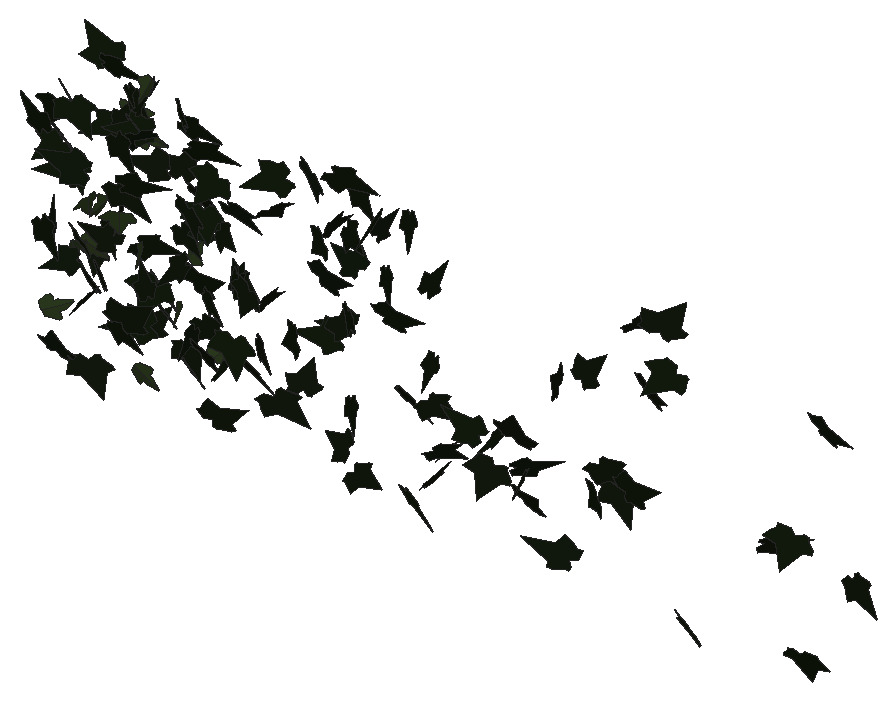
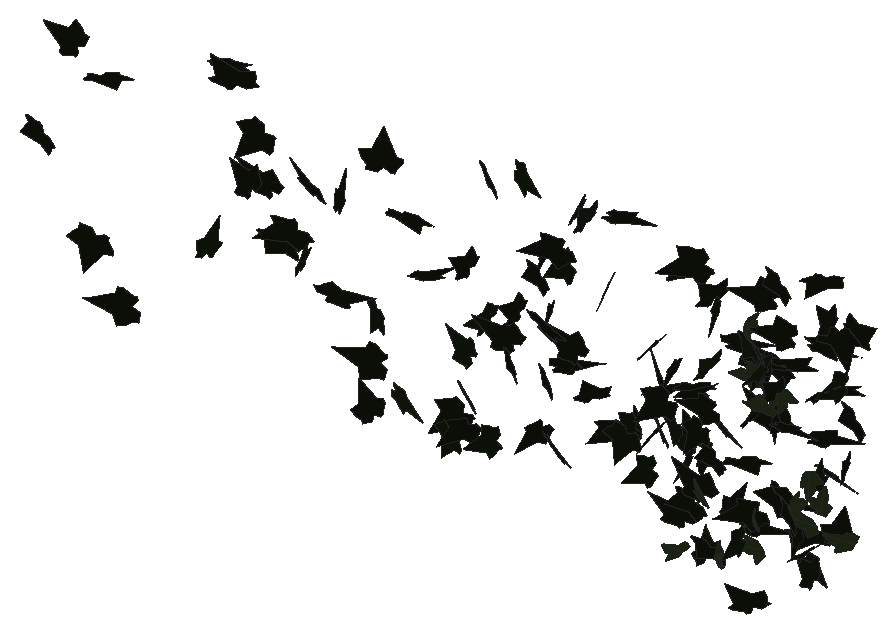
# SketchUp Ruby script. Lengths in inches.
U = 1.inch
M = Sketchup.active_model
def pt(a) = Geom::Point3d.new(a.map { |v| v * U })
def face(e, loops, mat)
  f = e.add_face(loops[0].map { |a| pt(a) })
  loops[1..].each { |l| e.add_face(l.map { |a| pt(a) }).erase! }
  f.material = f.back_material = mat if mat
  f
end
# faces: each face lists its corners as indices into pts; further lists are holes
def faces(e, pts, list, mat = nil) = list.each { |f| face(e, (f[0].is_a?(Array) ? f : [f]).map { |l| l.map { |i| pts[i] } }, mat) }
# xy, xz, yz: faces in a plane at the given z, y or x. An outline is a flat list of corners, or four numbers for a rectangle; further outlines are holes
def ring(l) = l.size == 4 ? [[l[0], l[1]], [l[2], l[1]], [l[2], l[3]], [l[0], l[3]]] : l.each_slice(2).to_a
def flat(e, list, mat, &to3) = list.each { |f| face(e, (f[0].is_a?(Array) ? f : [f]).map { |l| ring(l).map { |u, v| to3.(u, v) } }, mat) }
def xy(e, z, list, mat = nil) = flat(e, list, mat) { |x, y| [x, y, z] }
def xz(e, y, list, mat = nil) = flat(e, list, mat) { |x, z| [x, y, z] }
def yz(e, x, list, mat = nil) = flat(e, list, mat) { |y, z| [x, y, z] }
def lines(e, pts, list) = list.each { |a, b| e.add_line(pt(pts[a]), pt(pts[b])) }
# prism: a flat outline (further loops are holes) pulled along v
def prism(e, loops, v, mat = nil)
  f = face(e, loops, mat); d = Geom::Vector3d.new(v.map { |x| x * U })
  f.pushpull(f.normal.samedirection?(d) ? d.length : -d.length)
end
def box(e, o, s, mat = nil) = prism(e, [[o, [o[0] + s[0], o[1], o[2]], [o[0] + s[0], o[1] + s[1], o[2]], [o[0], o[1] + s[1], o[2]]]], [0, 0, s[2]], mat)
def at(x, y, z, deg = 0) = Geom::Transformation.translation(pt([x, y, z])) * Geom::Transformation.rotation(ORIGIN, Z_AXIS, deg.degrees)
def axes(o, x, y, z) = Geom::Transformation.new([*x, 0, *y, 0, *z, 0, *pt(o).to_a, 1])
def part(name) = M.definitions.add(name)
# library, detail: a bought-in or finely detailed component or shape, given as its bounding box
def library(name, o, s) = part(name).tap { |d| box(d.entities, o, s) }
def detail(e, o, s) = box(e.add_group.entities, o, s)
def put(e, d, t, mat = nil) = e.add_instance(d, t).tap { |i| i.material = mat if mat }
def group(e, t, mat = nil) = e.add_group.tap { |g| g.transformation = t; g.material = mat if mat }.entities
root = M.entities
M.materials.add("1026 AP 7946 SUNNY SIDE UP").color = [254, 231, 186]
M.materials.add("efeu1").color = [18, 25, 13]
M.materials.add("efeu2").color = [43, 57, 29]
c1 = part("ivyleaf_9")
p = [[1.54,2.16,1.25],[1.36,2.04,1.19],[-0.21,0.99,0.68],[-0.71,1.11,0.82],[-0.85,0.86,0.67],[-0.8,0.17,0.21],
  [-0.9,-0.01,0.1],[-0.67,-0.16,-0.02],[-0.08,-0.08,-0.05],[-0.03,-0.6,-0.4],[0.65,-0.88,-0.66],[0.83,-0.6,-0.49],
  [1.29,-0.42,-0.43],[1.8125,-0.07,-0.26],[1.21,0.44,0.15]]
faces(c1.entities,p,[[0,1,2,3,4,5,6,7,8,9,10,11,12,13,14]],"efeu1")
c2 = part("ivyleaf_10")
p = [[0,0.5,-0.03],[-0.0625,2.02,-0.43],[-0.19,2.01,-0.46],[-0.54,1.05,-0.29],[-0.52,0.625,-0.18],[-0.83,0.76,-0.28],
  [-1.16,0.64,-0.33],[-1.15,0.33,-0.24],[-0.77,-0.39,0.02],[-0.3,-0.51,0.16],[0.04,-0.48,0.23],[-0.02,2.01,-0.4375],
  [-0.06,2.01,-0.43],[0.04,-0.49,0.23],[0.67,-0.49,0.14],[1.38,0.36,-0.2],[1.375,0.51,-0.24],[0.81,0.65,-0.19],
  [0.62,0.59,-0.15],[0.6,1.09,-0.28],[0.5,1.23,-0.31]]
faces(c2.entities,p,[[0,1,2,3,4,5,6,7,8,9,10],[11,12,0,13,14,15,16,17,18,19,20]],"efeu2")
put(root,c1,axes([156.98,210.53,286.43],[-0.47696,-0.0723,0.34945],[-0.49379,-0.13528,-0.31941],[0.23295,-0.4348,0.03841]),"1026 AP 7946 SUNNY SIDE UP")
put(root,c1,axes([156.96,212.43,290.43],[-0.65372,-0.19497,-0.00524],[-0.03193,0.03396,0.47151],[-0.30497,0.41438,-0.03813]),"1026 AP 7946 SUNNY SIDE UP")
put(root,c1,axes([156.29,211.76,281.18],[0.15068,-0.21401,0.39414],[0.19777,-0.36304,-0.24301],[0.66207,0.15715,-0.01711]),"1026 AP 7946 SUNNY SIDE UP")
put(root,c1,axes([156.55,212.05,282.28],[-0.09183,-0.37678,0.07217],[-0.00305,-0.07274,-0.39311],[0.60323,-0.05773,0.009]),"1026 AP 7946 SUNNY SIDE UP")
put(root,c1,axes([156.81,209.09,284.39],[-0.06746,-0.14859,0.41575],[0.1899,0.38597,0.16155],[-0.65029,0.12813,0.00405]),"1026 AP 7946 SUNNY SIDE UP")
put(root,c1,axes([156.93,209.47,288.05],[-0.43996,-0.22259,0.17657],[-0.16855,-0.14092,-0.36694],[0.40962,-0.29705,0.03866]),"1026 AP 7946 SUNNY SIDE UP")
put(root,c1,axes([156.47,209.7,288.51],[0.53514,-0.28084,0.00143],[-0.02885,-0.0269,-0.45349],[0.44068,0.33928,-0.03142]),"1026 AP 7946 SUNNY SIDE UP")
put(root,c2,axes([156.85,212.1,284.22],[0.05882,-0.06243,0.38985],[0.14433,-0.36808,-0.07399],[0.58612,0.0969,-0.0209]),"1026 AP 7946 SUNNY SIDE UP")
put(root,c1,axes([157.3,212.36,287.67],[-0.55836,-0.03377,0.15532],[-0.22596,-0.06788,-0.36428],[0.09002,-0.37984,0.04898]),"1026 AP 7946 SUNNY SIDE UP")
put(root,c2,axes([157.02,211.03,284.94],[-0.12068,-0.38239,-0.10532],[0.04398,0.09642,-0.40114],[0.61995,-0.08127,0.00796]),"1026 AP 7946 SUNNY SIDE UP")
put(root,c1,axes([157.3,207.87,289.59],[0.10643,-0.08708,0.41704],[-0.33907,0.34336,0.1151],[-0.55673,-0.22576,0.00963]),"1026 AP 7946 SUNNY SIDE UP")
put(root,c1,axes([157.29,208.88,290.14],[0.45969,0.1171,-0.34721],[-0.46,-0.17227,-0.32345],[-0.32291,0.41211,-0.03352]),"1026 AP 7946 SUNNY SIDE UP")
put(root,c2,axes([157.16,210.14,283.16],[-0.15146,-0.31849,-0.23263],[-0.05871,-0.22214,0.34061],[-0.60943,0.10055,0.025]),"1026 AP 7946 SUNNY SIDE UP")
put(root,c1,axes([157.4,210.64,281.125],[-0.2473,0.28417,-0.22099],[0.13859,-0.19795,-0.33537],[-0.54401,-0.17961,0.01502]),"1026 AP 7946 SUNNY SIDE UP")
put(root,c2,axes([156.89,208.78,281.2],[0.21959,0.05592,-0.3699],[0.47428,0.19729,0.15353],[0.31955,-0.33125,0.02632]),"1026 AP 7946 SUNNY SIDE UP")
put(root,c2,axes([156.9,211.125,283],[-0.15781,-0.00986,-0.38759],[0.53061,-0.17465,-0.08905],[-0.26185,-0.34796,0.05313]),"1026 AP 7946 SUNNY SIDE UP")
put(root,c1,axes([157.32,211.83,283.62],[-0.15407,-0.05736,-0.45334],[0.68366,-0.10099,-0.08683],[-0.13713,-0.43904,0.07645]),"1026 AP 7946 SUNNY SIDE UP")
put(root,c1,axes([157.5,209.95,283.87],[0.40486,-0.27997,-0.16395],[0.22451,-0.08114,0.38846],[-0.45252,-0.29074,0.04605]),"1026 AP 7946 SUNNY SIDE UP")
put(root,c1,axes([157.8,210.69,282.3],[0.38912,-0.12408,-0.28524],[-0.42309,0.07341,-0.28193],[0.21828,0.36349,-0.03797]),"1026 AP 7946 SUNNY SIDE UP")
put(root,c1,axes([158.3,210.9,283.57],[-0.24504,0.13816,0.36682],[-0.46789,0.19583,-0.21176],[-0.37467,-0.33491,0.02455]),"1026 AP 7946 SUNNY SIDE UP")
put(root,c1,axes([158.27,208.62,283.81],[-0.58292,0.12185,0.08032],[-0.13464,-0.01432,-0.40003],[-0.18261,-0.37842,0.03855]),"1026 AP 7946 SUNNY SIDE UP")
put(root,c1,axes([157.56,209.14,290.48],[0.1385,-0.2344,0.36129],[0.14402,-0.34048,-0.25916],[0.64924,0.12553,-0.01958]),"1026 AP 7946 SUNNY SIDE UP")
put(root,c1,axes([157.77,209.3,287.59],[0.00105,-0.38969,-0.05874],[0.00218,0.0548,-0.40113],[0.61877,0.00047,0.00151]),"1026 AP 7946 SUNNY SIDE UP")
put(root,c2,axes([157.92,212.68,288.28],[0.61115,0.04956,-0.01353],[0.01222,0.04445,0.40146],[0.07981,-0.38636,0.04213]),"1026 AP 7946 SUNNY SIDE UP")
put(root,c1,axes([157.64,207.5,285.67],[-0.13472,-0.06788,-0.47571],[0.73317,-0.02084,-0.08616],[-0.01308,-0.4688,0.0699]),"1026 AP 7946 SUNNY SIDE UP")
put(root,c1,axes([158.23,211.51,288.37],[-0.15955,-0.07341,0.3889],[0.37642,0.29405,0.12678],[-0.47409,0.25818,-0.03022]),"1026 AP 7946 SUNNY SIDE UP")
put(root,c1,axes([158.22,207.64,280.35],[0.57197,-0.16928,0.12798],[-0.14963,0.09076,0.41178],[-0.29532,-0.37384,0.03925]),"1026 AP 7946 SUNNY SIDE UP")
put(root,c1,axes([157.77,211.34,290.89],[0.43355,-0.07208,0.29989],[0.41706,-0.12708,-0.29157],[0.22137,0.38059,-0.038]),"1026 AP 7946 SUNNY SIDE UP")
put(root,c1,axes([158.36,211.95,289.65],[0.45232,-0.35053,-0.09835],[-0.12695,0.05445,-0.46598],[0.55613,0.29753,-0.02638]),"1026 AP 7946 SUNNY SIDE UP")
put(root,c1,axes([159.29,207.76,288.46],[-0.44169,-0.17637,-0.35042],[-0.48797,-0.14052,0.33927],[-0.35096,0.41735,-0.0307]),"1026 AP 7946 SUNNY SIDE UP")
put(root,c2,axes([158.8125,212,283.01],[0.12533,-0.17766,0.35121],[0.26866,-0.29666,-0.20157],[0.54306,0.18777,0.01866]),"1026 AP 7946 SUNNY SIDE UP")
put(root,c1,axes([158.76,212.26,279.35],[-0.24949,-0.02099,0.41106],[0.61229,0.08869,0.16479],[-0.14167,0.42026,-0.01167]),"1026 AP 7946 SUNNY SIDE UP")
put(root,c1,axes([158.99,211.34,289.44],[-0.09333,0.32331,0.26054],[0.09219,-0.24437,0.33703],[0.63702,0.08273,-0.0106]),"1026 AP 7946 SUNNY SIDE UP")
put(root,c1,axes([158.87,211.97,283.25],[0.09768,0.09358,-0.42869],[0.1525,0.40694,0.11143],[0.65392,-0.10888,0.03805]),"1026 AP 7946 SUNNY SIDE UP")
put(root,c1,axes([159.03,207.58,291.3],[-0.11704,-0.34068,-0.2994],[0.13206,0.27677,-0.35716],[0.68961,-0.11082,0.01758]),"1026 AP 7946 SUNNY SIDE UP")
put(root,c1,axes([159.55,211.47,290.08],[-0.30208,0.18477,-0.35045],[-0.3728,0.24553,0.27592],[0.48302,0.30506,-0.00622]),"1026 AP 7946 SUNNY SIDE UP")
put(root,c1,axes([159.29,210.91,289.05],[0.50554,-0.04998,-0.26158],[-0.37961,0.08667,-0.33236],[0.14533,0.40023,0.04179]),"1026 AP 7946 SUNNY SIDE UP")
put(root,c1,axes([159.87,210.94,288.9],[-0.46343,0.0187,0.29618],[-0.44927,-0.07063,-0.29754],[0.05688,-0.40555,0.06303]),"1026 AP 7946 SUNNY SIDE UP")
put(root,c1,axes([159.47,210.08,286.16],[-0.17716,0.05385,-0.46499],[0.55483,-0.28329,-0.12713],[-0.45134,-0.36938,0.02623]),"1026 AP 7946 SUNNY SIDE UP")
put(root,c1,axes([159.43,212.09,281.89],[0.53175,-0.23609,-0.13661],[-0.20248,0.04399,-0.42301],[0.37337,0.36008,-0.03485]),"1026 AP 7946 SUNNY SIDE UP")
put(root,c1,axes([159.81,210.46,288.9375],[0.20341,0.36905,-0.12404],[-0.04412,-0.11991,-0.40336],[-0.60983,0.13177,-0.01219]),"1026 AP 7946 SUNNY SIDE UP")
put(root,c2,axes([159.68,211.34,290.71],[-0.05764,-0.21073,0.35169],[0.18287,-0.33486,-0.20134],[0.60541,0.08108,0.0943]),"1026 AP 7946 SUNNY SIDE UP")
put(root,c1,axes([159.625,207.84,280.26],[-0.26815,-0.30677,-0.30622],[0.24472,0.25142,-0.35994],[0.62345,-0.23063,0.00958]),"1026 AP 7946 SUNNY SIDE UP")
put(root,c2,axes([159.39,211.18,288.48],[0.07586,-0.02695,0.40589],[0.57939,0.1463,-0.0353],[-0.22407,0.36916,0.04613]),"1026 AP 7946 SUNNY SIDE UP")
put(root,c1,axes([160.64,210.09,281.13],[-0.50567,-0.06402,0.34178],[-0.49223,-0.11721,-0.33623],[0.2014,-0.4472,0.03635]),"1026 AP 7946 SUNNY SIDE UP")
put(root,c1,axes([159.73,213.55,288.05],[0.20859,0.0152,-0.38255],[0.52624,0.16678,0.13115],[0.25444,-0.35741,0.04238]),"1026 AP 7946 SUNNY SIDE UP")
put(root,c2,axes([160.35,208.77,286.37],[-0.49706,-0.25232,0.0011],[0.02723,-0.02569,-0.41562],[0.39583,-0.31508,0.02997]),"1026 AP 7946 SUNNY SIDE UP")
put(root,c2,axes([160.45,212.2,280.84],[0.09775,-0.06391,0.3986],[0.30975,-0.33407,-0.09133],[0.53384,0.20554,-0.01999]),"1026 AP 7946 SUNNY SIDE UP")
put(root,c1,axes([160.3,208.55,281.77],[0.12244,-0.03234,-0.4473],[0.68057,0.0519,0.07632],[0.07163,-0.43787,0.03947]),"1026 AP 7946 SUNNY SIDE UP")
put(root,c1,axes([160.39,208.71,287.63],[-0.06815,-0.11326,-0.46432],[0.6415,0.2062,-0.09272],[0.34789,-0.4024,0.08001]),"1026 AP 7946 SUNNY SIDE UP")
put(root,c2,axes([160.89,212.5,283.22],[0.41093,-0.27679,-0.12134],[0.15812,-0.06447,0.39075],[-0.44476,-0.27865,0.02681]),"1026 AP 7946 SUNNY SIDE UP")
put(root,c1,axes([161.26,210.41,281.73],[0.34672,-0.33138,0.12282],[-0.07154,0.1149,0.40994],[-0.55013,-0.22379,0.02409]),"1026 AP 7946 SUNNY SIDE UP")
put(root,c1,axes([161.77,209.69,288.49],[-0.30476,0.03665,0.38893],[-0.59498,-0.04476,-0.19601],[0.03665,-0.42183,0.05208]),"1026 AP 7946 SUNNY SIDE UP")
put(root,c2,axes([160.95,209.24,279.71],[-0.24456,0.0736,-0.36602],[0.46887,-0.1951,-0.17704],[-0.32618,-0.33564,0.01993]),"1026 AP 7946 SUNNY SIDE UP")
put(root,c1,axes([161.17,212.36,286.18],[0.58114,-0.06621,-0.1475],[-0.23212,-0.01936,-0.38447],[0.08588,0.39574,-0.0411]),"1026 AP 7946 SUNNY SIDE UP")
put(root,c1,axes([161.01,211.72,284.72],[-0.09259,-0.07439,-0.39659],[0.60568,0.05945,-0.07226],[0.11157,-0.38446,0.06317]),"1026 AP 7946 SUNNY SIDE UP")
put(root,c1,axes([161.48,209.54,283.49],[-0.52684,-0.33177,-0.02183],[0.05563,-0.00835,-0.48477],[0.51959,-0.33551,0.02977]),"1026 AP 7946 SUNNY SIDE UP")
put(root,c1,axes([161.1,207.68,290.4],[-0.1284,-0.07617,-0.45184],[0.69835,0.0093,-0.08688],[0.03653,-0.44561,0.07274]),"1026 AP 7946 SUNNY SIDE UP")
put(root,c1,axes([161.7,210.68,290.6],[0.34088,-0.12733,-0.344],[-0.46087,0.15863,-0.25798],[0.31965,0.36449,-0.0051]),"1026 AP 7946 SUNNY SIDE UP")
put(root,c1,axes([161.83,211.01,280.27],[-0.30579,-0.11451,-0.35275],[0.51265,0.1097,-0.22834],[0.24166,-0.37761,0.03804]),"1026 AP 7946 SUNNY SIDE UP")
put(root,c1,axes([162.4,207.87,284.17],[-0.22349,-0.25493,0.29256],[0.17981,0.26228,0.30152],[-0.57427,0.18133,-0.01945]),"1026 AP 7946 SUNNY SIDE UP")
put(root,c1,axes([161.81,211.47,282.83],[-0.03365,-0.04358,0.47663],[0.53114,-0.31989,-0.01681],[0.50239,0.33528,0.04969]),"1026 AP 7946 SUNNY SIDE UP")
put(root,c1,axes([162.24,210.67,279.62],[0.47209,-0.2333,-0.19638],[0.26897,-0.08726,0.38978],[-0.38836,-0.34404,0.03123]),"1026 AP 7946 SUNNY SIDE UP")
put(root,c1,axes([162.85,209.47,284.8],[-0.61141,0.19895,-0.13854],[0.15423,-0.10436,-0.44806],[-0.34575,-0.39836,0.04512]),"1026 AP 7946 SUNNY SIDE UP")
put(root,c1,axes([162.12,206.97,289.1],[0.29812,0.03645,0.39496],[0.60347,0.01458,-0.19698],[-0.04602,0.42727,-0.02445]),"1026 AP 7946 SUNNY SIDE UP")
put(root,c1,axes([162.31,206.51,283.5],[-0.24563,0.05671,0.46277],[0.61667,-0.21985,0.16793],[0.35478,0.42139,0.02852]),"1026 AP 7946 SUNNY SIDE UP")
put(root,c2,axes([162.78,211.58,280.02],[0.25159,0.15526,-0.3434],[0.26858,0.29162,0.22551],[0.51346,-0.22861,0.05031]),"1026 AP 7946 SUNNY SIDE UP")
put(root,c1,axes([163.36,210.52,286.01],[-0.39898,-0.34593,-0.01741],[-0.02742,-0.00573,0.44179],[-0.54375,0.25411,-0.0095]),"1026 AP 7946 SUNNY SIDE UP")
put(root,c1,axes([162.92,210.62,286.68],[-0.248,-0.36436,-0.13307],[0.12968,0.10231,-0.40698],[0.59277,-0.17482,0.03336]),"1026 AP 7946 SUNNY SIDE UP")
put(root,c1,axes([162.84,209.8,287.0625],[0.10245,-0.40694,0.25071],[0.06959,-0.2417,-0.42595],[0.74419,0.07862,0.00531]),"1026 AP 7946 SUNNY SIDE UP")
put(root,c1,axes([162.79,210.78,281.75],[-0.0445,-0.06057,-0.435],[0.62363,0.15114,-0.04888],[0.2455,-0.39492,0.04531]),"1026 AP 7946 SUNNY SIDE UP")
put(root,c1,axes([163.32,210.29,283.26],[0.39798,-0.26799,-0.21284],[-0.2645,0.12204,-0.37745],[0.46,0.30204,-0.03289]),"1026 AP 7946 SUNNY SIDE UP")
put(root,c1,axes([163.51,208.64,289.375],[-0.2633,-0.11343,0.44636],[0.47489,0.31391,0.20644],[-0.52138,0.34321,-0.03738]),"1026 AP 7946 SUNNY SIDE UP")
put(root,c1,axes([163.26,211.83,286.42],[0.69883,0.01112,0.00539],[0.0096,-0.03795,-0.45653],[-0.01672,0.44284,-0.03665]),"1026 AP 7946 SUNNY SIDE UP")
put(root,c1,axes([163.66,213.69,285.65],[0.26052,0.38491,0.09461],[0.07962,0.07574,-0.43094],[-0.61631,0.17249,-0.01568]),"1026 AP 7946 SUNNY SIDE UP")
put(root,c1,axes([163.84,208.84,282.5625],[-0.08736,0.05152,-0.42564],[0.39097,-0.3306,-0.07879],[-0.5257,-0.25443,0.01213]),"1026 AP 7946 SUNNY SIDE UP")
put(root,c1,axes([164.5625,210.54,284.21],[-0.04022,0.17931,0.39924],[-0.06364,0.38444,-0.18424],[-0.66695,-0.0475,-0.00649]),"1026 AP 7946 SUNNY SIDE UP")
put(root,c1,axes([164.4375,209.79,286.6875],[0.21583,-0.18172,-0.34754],[-0.33637,0.25964,-0.23295],[0.49815,0.25405,-0.00672]),"1026 AP 7946 SUNNY SIDE UP")
put(root,c1,axes([164.0625,208.67,290.61],[0.58756,0.127,0.2591],[0.40047,0.02361,-0.40312],[-0.18708,0.44941,-0.0492]),"1026 AP 7946 SUNNY SIDE UP")
put(root,c1,axes([164.48,210.77,284.32],[0.30408,-0.24135,-0.2936],[-0.22856,0.24532,-0.31573],[0.53915,0.24013,0.03175]),"1026 AP 7946 SUNNY SIDE UP")
put(root,c1,axes([165.2,208.54,289.77],[-0.39779,-0.34776,0.19419],[-0.11414,-0.1815,-0.44177],[0.61292,-0.25949,0.04377]),"1026 AP 7946 SUNNY SIDE UP")
put(root,c1,axes([164.85,208.05,282.35],[0.59403,-0.16828,-0.21791],[0.33173,-0.04105,0.4235],[-0.26381,-0.43055,0.04187]),"1026 AP 7946 SUNNY SIDE UP")
put(root,c1,axes([164.99,208.66,279.29],[-0.09695,0.0436,0.42691],[0.60634,-0.15211,0.07475],[0.24726,0.39011,-0.01591]),"1026 AP 7946 SUNNY SIDE UP")
put(root,c1,axes([165.68,209.04,284.99],[-0.08943,0.22879,0.3665],[0.04693,-0.35459,0.23864],[0.66171,0.05607,0.03261]),"1026 AP 7946 SUNNY SIDE UP")
put(root,c1,axes([165.85,210.52,283.77],[0.15381,0.23255,0.3607],[0.26252,0.30693,-0.25726],[-0.60465,0.19242,-0.01994]),"1026 AP 7946 SUNNY SIDE UP")
put(root,c1,axes([165.79,209.58,281.55],[0.60021,-0.19192,0.02646],[0.01212,-0.04405,-0.43885],[0.30445,0.38011,-0.03468]),"1026 AP 7946 SUNNY SIDE UP")
put(root,c1,axes([166.37,207.35,282.36],[0.01232,0.29681,0.3049],[0.01264,0.29417,-0.30415],[-0.65709,0.01122,-0.00014]),"1026 AP 7946 SUNNY SIDE UP")
put(root,c1,axes([166.84,207.5,283.82],[-0.21201,-0.45538,-0.07921],[0.07545,0.06315,-0.48806],[0.72158,-0.1404,0.02776]),"1026 AP 7946 SUNNY SIDE UP")
put(root,c1,axes([166.99,208.21,285.69],[-0.08743,-0.36188,0.29092],[-0.05319,-0.28253,-0.37876],[0.72181,-0.06465,0.00732]),"1026 AP 7946 SUNNY SIDE UP")
put(root,c1,axes([166.79,209.1,283],[0.02683,-0.04256,-0.43843],[0.64845,-0.11038,0.02778],[-0.17688,-0.41112,0.03533]),"1026 AP 7946 SUNNY SIDE UP")
put(root,c1,axes([168.51,208.39,291.02],[-0.56226,-0.12358,0.26125],[-0.35084,-0.12849,-0.38829],[0.27305,-0.41955,0.03906]),"1026 AP 7946 SUNNY SIDE UP")
put(root,c1,axes([168.48,208.02,281.72],[-0.04938,-0.17817,-0.44182],[0.28917,0.38885,-0.17844],[0.66894,-0.18124,0.04452]),"1026 AP 7946 SUNNY SIDE UP")
put(root,c1,axes([168.73,210.44,285.94],[0.11039,-0.06812,0.46838],[0.47635,-0.33961,-0.10251],[0.54453,0.31089,-0.00528]),"1026 AP 7946 SUNNY SIDE UP")
put(root,c1,axes([169.09,209.35,291.01],[0.09645,-0.35358,0.32685],[0.06865,-0.31639,-0.37145],[0.74594,0.07484,-0.00808]),"1026 AP 7946 SUNNY SIDE UP")
put(root,c1,axes([169.22,210.73,290.42],[0.09793,0.02972,-0.44758],[0.42859,0.33984,0.06616],[0.53437,-0.27801,0.02896]),"1026 AP 7946 SUNNY SIDE UP")
put(root,c1,axes([170.23,210.68,286.77],[-0.14883,0.20014,0.40113],[-0.38532,0.3045,-0.22148],[-0.56853,-0.25877,0.0451]),"1026 AP 7946 SUNNY SIDE UP")
put(root,c1,axes([169.82,208,282.6],[-0.3843,-0.08842,0.32333],[0.42419,0.1666,0.26532],[-0.28935,0.36166,-0.04048]),"1026 AP 7946 SUNNY SIDE UP")
put(root,c1,axes([170.37,209.33,284.33],[-0.32482,-0.01071,0.41109],[-0.59115,-0.14602,-0.20536],[0.21128,-0.42501,0.05742]),"1026 AP 7946 SUNNY SIDE UP")
put(root,c1,axes([169.57,211.5625,289.47],[-0.09686,-0.05977,-0.42188],[0.64928,0.01336,-0.06598],[0.03498,-0.41358,0.05636]),"1026 AP 7946 SUNNY SIDE UP")
put(root,c1,axes([169.9,209.38,288.88],[0.16793,0.22561,0.40785],[0.30423,0.34425,-0.25468],[-0.64677,0.22051,-0.0139]),"1026 AP 7946 SUNNY SIDE UP")
put(root,c1,axes([170.35,211.85,287.79],[-0.05728,0.01897,0.4331],[0.40713,0.33353,0.00956],[-0.52143,0.25833,-0.04011]),"1026 AP 7946 SUNNY SIDE UP")
put(root,c1,axes([170.3,212.37,285.85],[-0.21093,0.00302,-0.41589],[0.6085,-0.12025,-0.1341],[-0.18088,-0.40807,0.03385]),"1026 AP 7946 SUNNY SIDE UP")
put(root,c1,axes([171.09,209.1,285.24],[-0.43581,0.29768,0.20138],[-0.24921,0.11633,-0.41694],[-0.49983,-0.31755,0.0323]),"1026 AP 7946 SUNNY SIDE UP")
put(root,c1,axes([170.73,206.37,285.69],[-0.07497,-0.08453,0.47301],[-0.18605,-0.44478,-0.09952],[0.7109,-0.12532,0.02384]),"1026 AP 7946 SUNNY SIDE UP")
put(root,c1,axes([171.41,208.6,280.35],[-0.34577,0.01641,-0.40658],[-0.6026,0.10101,0.22484],[0.15109,0.44043,-0.0337]),"1026 AP 7946 SUNNY SIDE UP")
put(root,c1,axes([170.9,209.34,289.26],[0.26305,-0.25886,-0.36682],[-0.37783,0.26361,-0.31349],[0.57777,0.29024,-0.038]),"1026 AP 7946 SUNNY SIDE UP")
put(root,c1,axes([171.1875,207.4,289.64],[-0.09653,-0.16967,0.40294],[-0.09705,-0.38844,-0.18539],[0.66473,-0.08135,0.03144]),"1026 AP 7946 SUNNY SIDE UP")
put(root,c1,axes([171.21,208.93,285.96],[0.19417,-0.11932,-0.3978],[0.49484,-0.22382,0.17393],[-0.3971,-0.33725,0.02223]),"1026 AP 7946 SUNNY SIDE UP")
put(root,c1,axes([171.75,211.52,281.57],[0.58663,-0.18786,0.08067],[0.08266,-0.07131,-0.42883],[0.30984,0.37471,-0.03834]),"1026 AP 7946 SUNNY SIDE UP")
put(root,c1,axes([172.02,208.12,282.71],[-0.22612,-0.00359,-0.40932],[0.6024,-0.11326,-0.14246],[-0.16561,-0.40707,0.04068]),"1026 AP 7946 SUNNY SIDE UP")
put(root,c1,axes([171.85,210.4375,285.33],[0.14922,-0.07026,0.44151],[0.58429,-0.21471,-0.12218],[0.35465,0.3833,0.01552]),"1026 AP 7946 SUNNY SIDE UP")
put(root,c1,axes([172.62,207.63,280.11],[0.08311,-0.10979,-0.43889],[-0.18662,0.40897,-0.12154],[0.66513,0.12847,0.02074]),"1026 AP 7946 SUNNY SIDE UP")
put(root,c1,axes([173.07,211.72,283.33],[-0.44611,0.07029,-0.32575],[0.45578,-0.13371,-0.29895],[-0.22871,-0.40355,0.03962]),"1026 AP 7946 SUNNY SIDE UP")
put(root,c1,axes([173.29,208.11,291.12],[-0.41635,0.1991,-0.35612],[0.36969,-0.25896,-0.33959],[-0.50864,-0.35118,0.04468]),"1026 AP 7946 SUNNY SIDE UP")
put(root,c1,axes([173.17,211.43,281.68],[-0.01328,-0.09668,-0.43034],[0.01609,0.41709,-0.09735],[0.67316,-0.01187,-0.00616]),"1026 AP 7946 SUNNY SIDE UP")
put(root,c1,axes([174.22,210,287.52],[-0.08817,-0.04116,0.45798],[0.44041,0.34598,0.07138],[-0.54716,0.28511,-0.01635]),"1026 AP 7946 SUNNY SIDE UP")
put(root,c1,axes([174.14,208.96,291.08],[-0.32556,0.01866,-0.40908],[0.59849,-0.12029,-0.21092],[-0.18093,-0.43147,0.03839]),"1026 AP 7946 SUNNY SIDE UP")
put(root,c1,axes([174.62,210.52,280.39],[0.10567,0.32143,0.28686],[0.08835,0.27086,-0.33671],[-0.66094,0.0876,0.00085]),"1026 AP 7946 SUNNY SIDE UP")
put(root,c1,axes([174.81,209.7,280.91],[0.44691,0.28778,0.21185],[0.26203,0.12137,-0.41485],[-0.48888,0.32813,-0.02869]),"1026 AP 7946 SUNNY SIDE UP")
put(root,c1,axes([176.77,211.07,281.67],[-0.4671,0.24587,-0.21257],[0.19077,-0.17631,-0.39474],[-0.4688,-0.31673,0.05117]),"1026 AP 7946 SUNNY SIDE UP")
put(root,c1,axes([176.76,206.8,281.45],[0.16021,0.41381,0.11738],[-0.09034,-0.10048,0.4373],[0.66783,-0.11286,0.03099]),"1026 AP 7946 SUNNY SIDE UP")
put(root,c1,axes([177.27,204.96,282.01],[0.44563,-0.36985,0.07199],[0.03787,-0.07211,-0.47978],[0.59125,0.28338,-0.02353]),"1026 AP 7946 SUNNY SIDE UP")
put(root,c1,axes([178.85,207.09,284.23],[-0.42755,-0.32454,-0.06651],[-0.09634,-0.03033,0.4351],[-0.51074,0.2774,-0.02639]),"1026 AP 7946 SUNNY SIDE UP")
put(root,c1,axes([178.55,210.35,279.88],[0.61169,-0.12986,-0.16127],[0.25575,-0.00163,0.41974],[-0.19055,-0.41905,0.04566]),"1026 AP 7946 SUNNY SIDE UP")
put(root,c1,axes([178.86,209.65,281.64],[0.28549,0.33552,-0.27319],[0.14533,0.25261,0.39312],[0.65848,-0.20122,0.03168]),"1026 AP 7946 SUNNY SIDE UP")
put(root,c1,axes([180.57,207.59,282.36],[-0.21679,0.16502,-0.41823],[-0.46968,0.27736,0.22177],[0.50607,0.32811,0.02666]),"1026 AP 7946 SUNNY SIDE UP")
put(root,c1,axes([181.64,204.64,284.83],[-0.62515,-0.20986,-0.11795],[0.18749,0.01583,-0.46117],[0.32477,-0.4131,0.03921]),"1026 AP 7946 SUNNY SIDE UP")
put(root,c1,axes([181.82,208.3125,286.79],[0.04486,0.11635,0.47767],[-0.25561,-0.43375,0.12008],[0.70581,-0.16448,0.01312]),"1026 AP 7946 SUNNY SIDE UP")
put(root,c1,axes([182.67,204.56,286.57],[0.67353,-0.13544,0.12635],[-0.15027,0.10261,0.4583],[-0.24583,-0.4338,0.06603]),"1026 AP 7946 SUNNY SIDE UP")
put(root,c1,axes([182.67,208.76,287.25],[-0.26264,0.30668,0.32502],[0.27117,-0.26281,0.35768],[0.63435,0.23932,-0.01833]),"1026 AP 7946 SUNNY SIDE UP")
put(root,c1,axes([184.05,206.05,281.12],[-0.21009,0.06828,0.4466],[-0.67687,0.06572,-0.14709],[-0.13118,-0.44848,0.0437]),"1026 AP 7946 SUNNY SIDE UP")
put(root,c1,axes([184.17,207.66,283.03],[-0.07838,-0.13393,0.45658],[-0.07476,-0.44269,-0.14566],[0.72531,-0.0601,0.03433]),"1026 AP 7946 SUNNY SIDE UP")
put(root,c1,axes([184.26,209.84,289.69],[0.36817,0.34529,0.24225],[0.2272,0.1836,-0.42846],[-0.6145,0.27476,-0.01327]),"1026 AP 7946 SUNNY SIDE UP")
put(root,c1,axes([184.44,207.67,284.53],[-0.00459,-0.02274,-0.48114],[0.45147,0.36839,-0.01818],[0.58006,-0.2869,0.01034]),"1026 AP 7946 SUNNY SIDE UP")
put(root,c1,axes([184.9375,209.74,287.08],[0.09254,-0.17766,0.45659],[0.30545,-0.40013,-0.19372],[0.68747,0.2017,0.02461]),"1026 AP 7946 SUNNY SIDE UP")
put(root,c1,axes([185.21,207.67,283.8],[-0.36452,-0.16537,-0.38475],[0.56163,0.12404,-0.28497],[0.30874,-0.42088,0.06414]),"1026 AP 7946 SUNNY SIDE UP")
put(root,c1,axes([186.41,208.73,290.63],[-0.40652,0.01373,0.416],[0.63199,-0.03933,0.2663],[0.0637,0.4778,0.01278]),"1026 AP 7946 SUNNY SIDE UP")
put(root,c1,axes([186.77,206.27,284.87],[0.03835,0.04008,0.46661],[0.5126,-0.31743,0.00901],[0.49793,0.32369,-0.04521]),"1026 AP 7946 SUNNY SIDE UP")
put(root,c1,axes([188.38,207.11,290.13],[-0.6428,-0.1886,0.10145],[-0.10603,-0.08986,-0.46121],[0.31812,-0.41104,0.05126]),"1026 AP 7946 SUNNY SIDE UP")
put(root,c1,axes([189.32,211.5,281.2],[0.18499,0.31814,-0.33059],[0.13834,0.31103,0.35074],[0.69899,-0.14575,0.01808]),"1026 AP 7946 SUNNY SIDE UP")
put(root,c1,axes([190.4,205.46,280.56],[0.46925,-0.36279,-0.05964],[0.09711,-0.0213,0.48255],[-0.56893,-0.30286,0.03318]),"1026 AP 7946 SUNNY SIDE UP")
put(root,c1,axes([194.66,206.92,280.28],[0.64927,0.13122,-0.19982],[-0.26864,-0.1023,-0.44487],[-0.25327,0.44491,-0.04039]),"1026 AP 7946 SUNNY SIDE UP")
put(root,c1,axes([194.42,208.38,289.33],[0.25462,-0.18023,0.42243],[0.41699,-0.31415,-0.25136],[0.56941,0.31066,-0.00482]),"1026 AP 7946 SUNNY SIDE UP")
put(root,c1,axes([195.46,205.44,286.32],[-0.49448,-0.35273,-0.03303],[0.06953,0.00075,-0.48567],[0.55228,-0.3159,0.03157]),"1026 AP 7946 SUNNY SIDE UP")
put(root,c1,axes([196.97,207.23,284.12],[-0.11233,-0.10344,-0.4784],[0.74105,0.04454,-0.08476],[0.09554,-0.46714,0.09496]),"1026 AP 7946 SUNNY SIDE UP")
